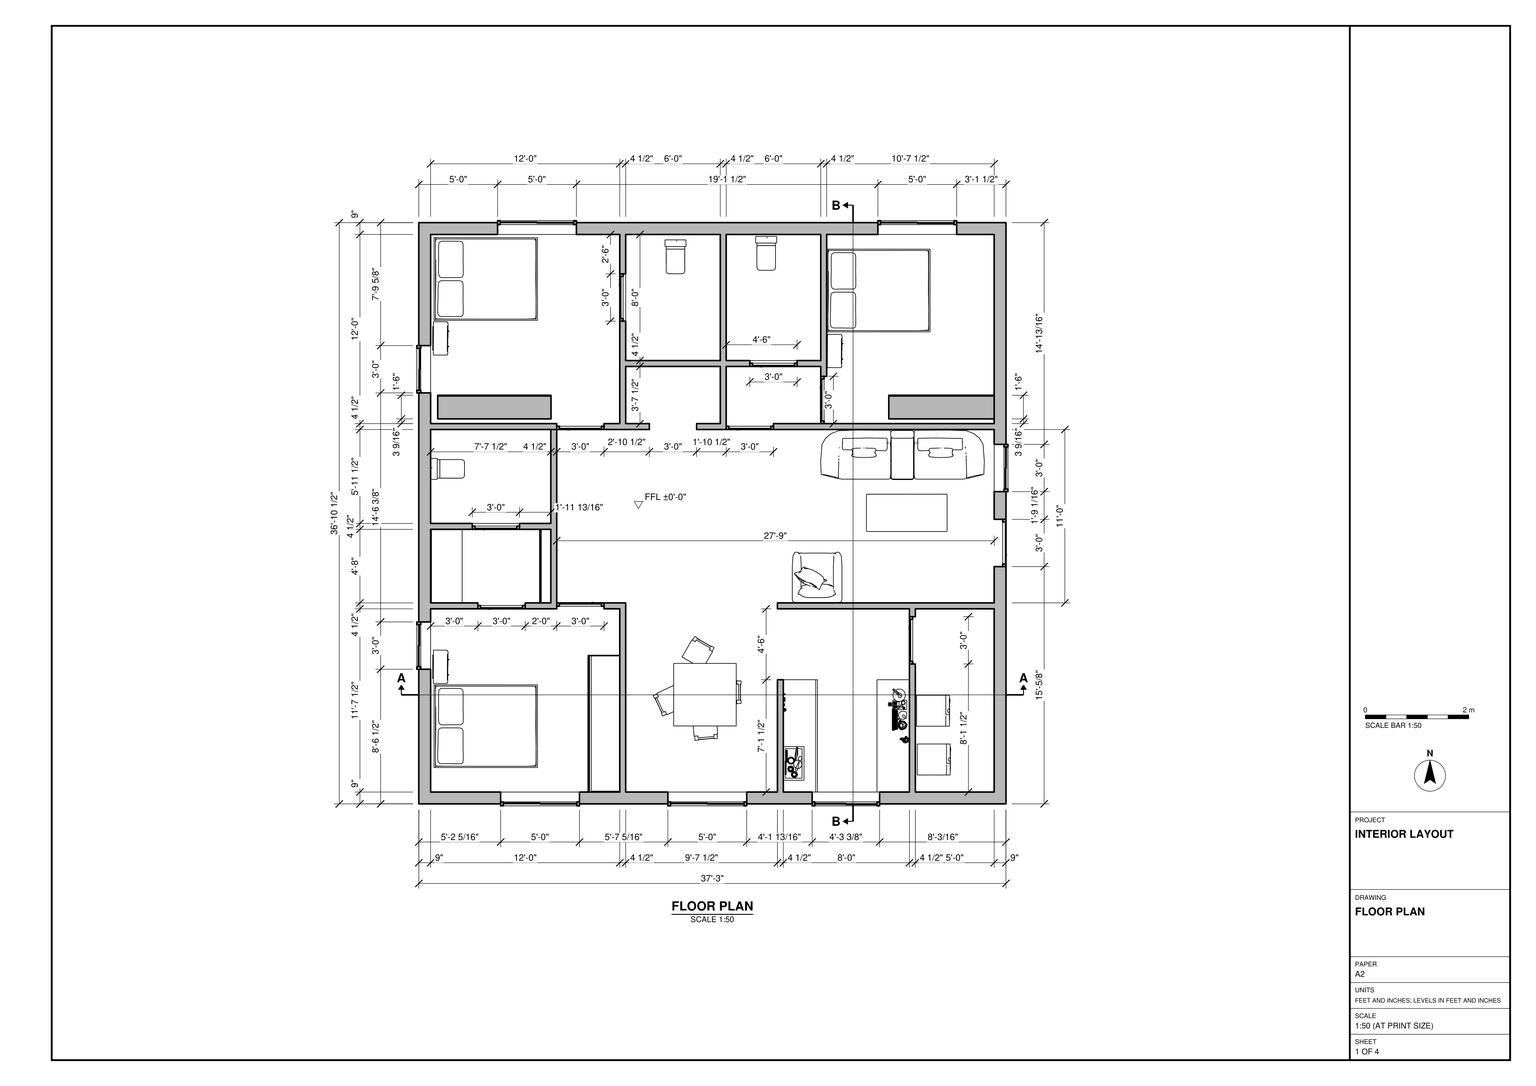
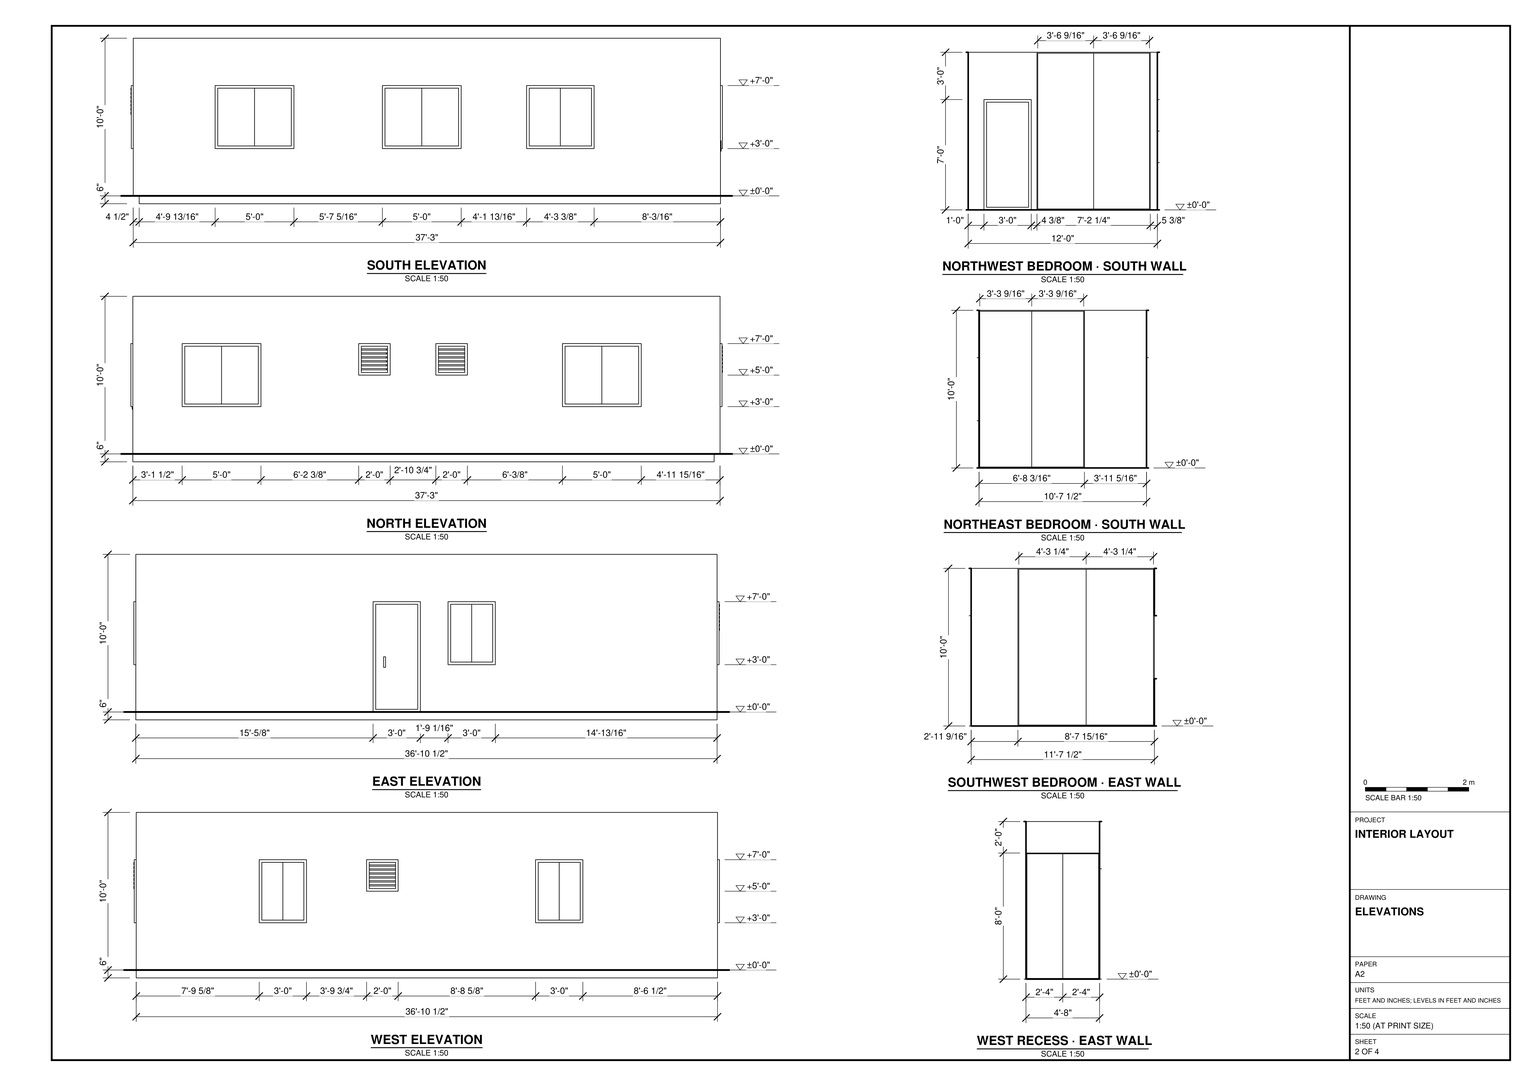
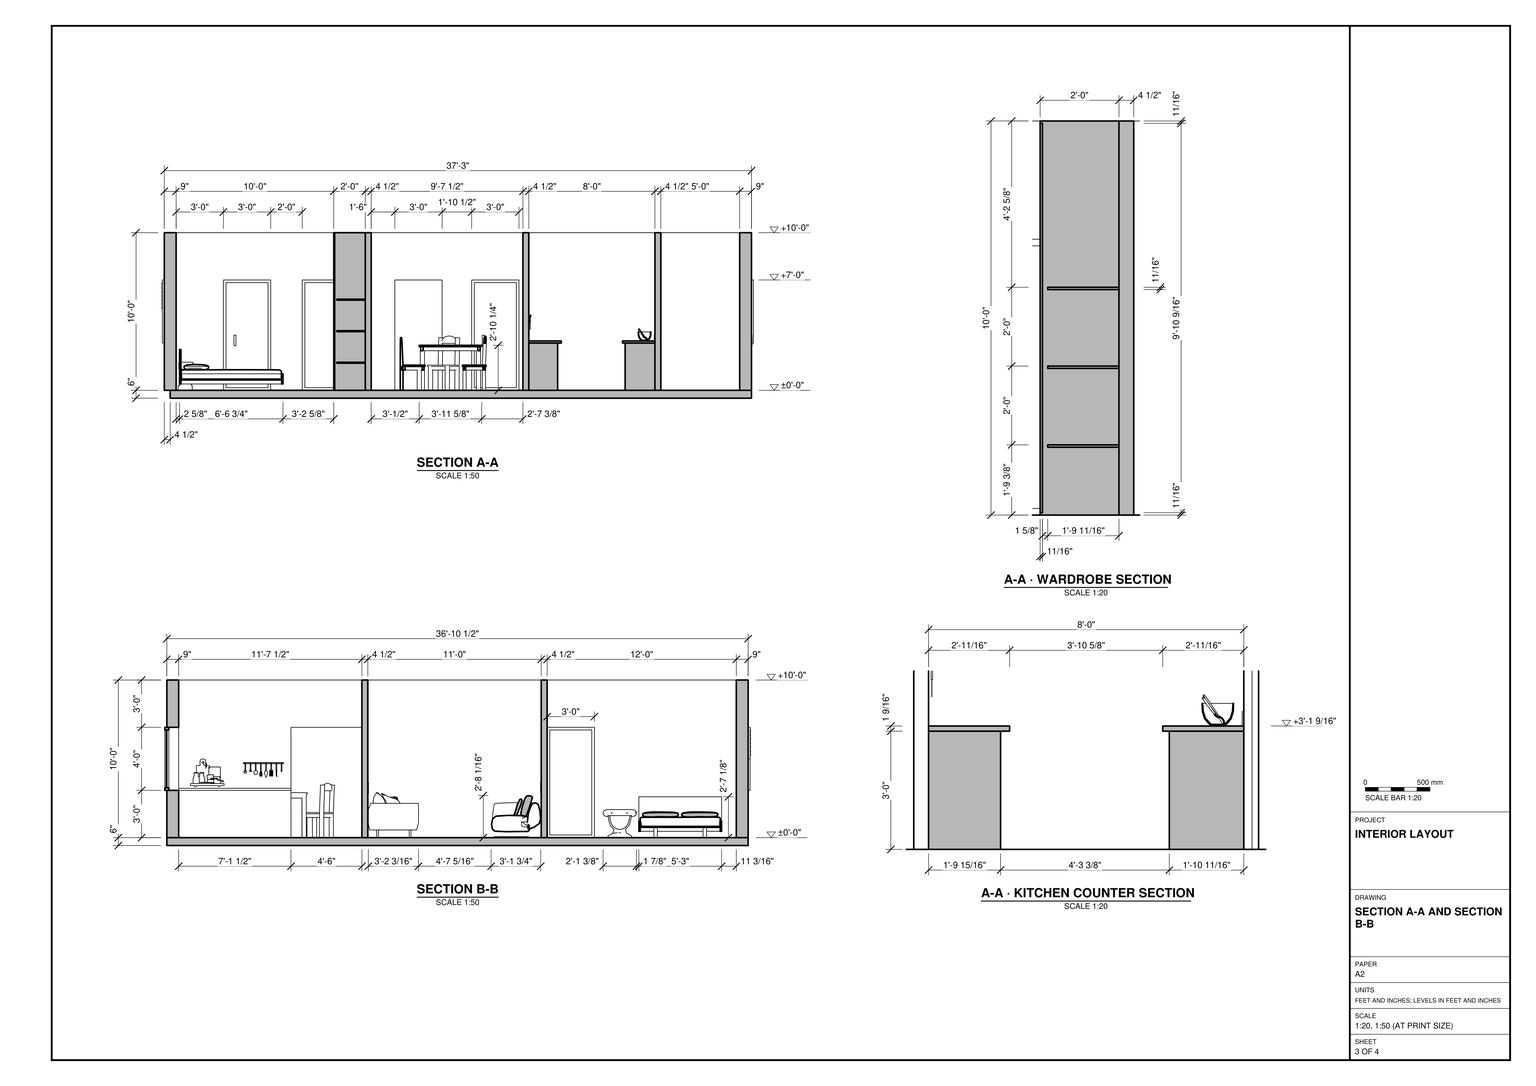
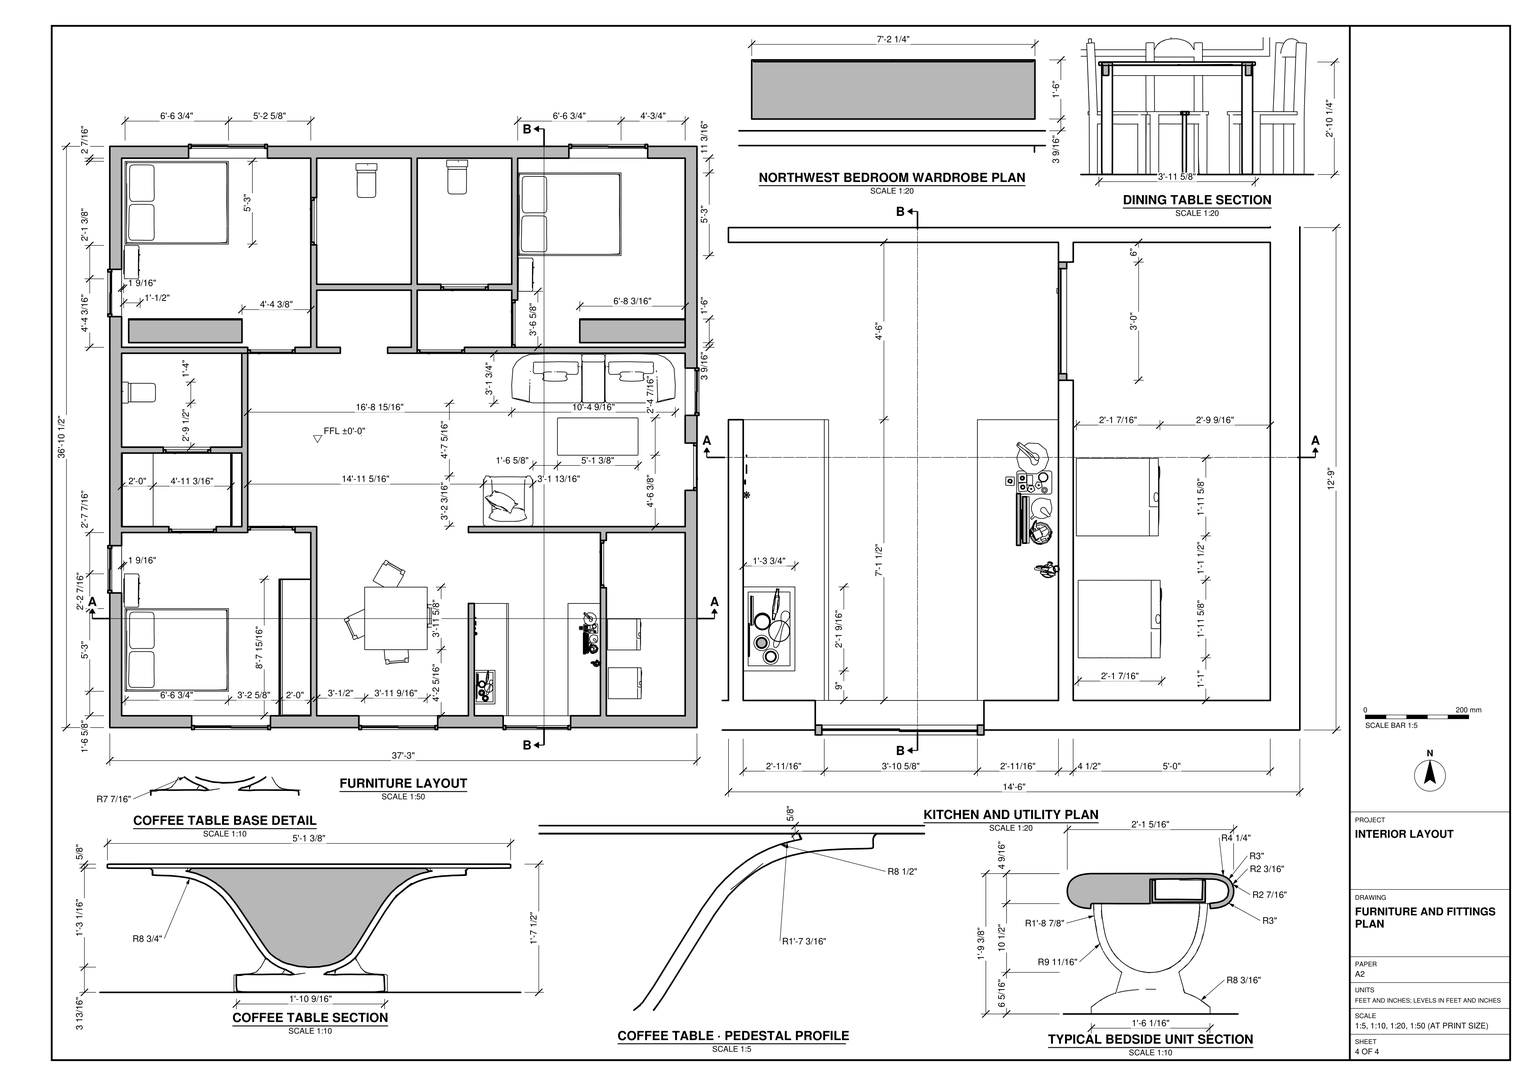
Build the single-storey interior shown in task_files/diagram_01.pdf. Work in feet and inches. Orient the plan with north at the top, east–west along X and north–south along Y. The overall model extents are 37'-6 5/16" along X, 37'-1 13/16" along Y and 10'-6" vertically. Set the finished floor at ±0'-0", with the 6" floor slab below it and the wall tops 10'-0" above it.

Use the plan to lay out the 9" exterior walls and 4 1/2" partitions. Place the bedrooms in the northwest, northeast and southwest corners. Fit the toilet compartments and west recess around the central living space, keeping the passages and doorways as drawn. Use the elevations to position the east entrance, windows and high-level vents.

Furnish the bedrooms with beds, bedside furniture and fitted wardrobes. Follow the interior elevations for the wardrobe widths and the section for the southwest wardrobe shelves. Arrange the sofa, low table and armchair in the eastern living area. Place the dining table and chairs south of the living space, beside the kitchen. Model the two facing kitchen counters with the aisle between them and place the appliances in the adjoining utility space. Decor and loose items, including appliances and kitchen utensils, may be any suitable library components.

Keep the slab, walls, and each furniture or joinery piece in separate groups or components, and use components for repeated parts. Save one SketchUp model as output_files/three_bedroom_interior_with_built_in_wardrobes.skp.

# SketchUp Ruby script. Lengths in inches.
U = 1.inch
M = Sketchup.active_model
def pt(a) = Geom::Point3d.new(a.map { |v| v * U })
def face(e, loops, mat)
  f = e.add_face(loops[0].map { |a| pt(a) })
  loops[1..].each { |l| e.add_face(l.map { |a| pt(a) }).erase! }
  f.material = f.back_material = mat if mat
  f
end
# faces: each face lists its corners as indices into pts; further lists are holes
def faces(e, pts, list, mat = nil) = list.each { |f| face(e, (f[0].is_a?(Array) ? f : [f]).map { |l| l.map { |i| pts[i] } }, mat) }
# xy, xz, yz: faces in a plane at the given z, y or x. An outline is a flat list of corners, or four numbers for a rectangle; further outlines are holes
def ring(l) = l.size == 4 ? [[l[0], l[1]], [l[2], l[1]], [l[2], l[3]], [l[0], l[3]]] : l.each_slice(2).to_a
def flat(e, list, mat, &to3) = list.each { |f| face(e, (f[0].is_a?(Array) ? f : [f]).map { |l| ring(l).map { |u, v| to3.(u, v) } }, mat) }
def xy(e, z, list, mat = nil) = flat(e, list, mat) { |x, y| [x, y, z] }
def xz(e, y, list, mat = nil) = flat(e, list, mat) { |x, z| [x, y, z] }
def yz(e, x, list, mat = nil) = flat(e, list, mat) { |y, z| [x, y, z] }
def lines(e, pts, list) = list.each { |a, b| e.add_line(pt(pts[a]), pt(pts[b])) }
# prism: a flat outline (further loops are holes) pulled along v
def prism(e, loops, v, mat = nil)
  f = face(e, loops, mat); d = Geom::Vector3d.new(v.map { |x| x * U })
  f.pushpull(f.normal.samedirection?(d) ? d.length : -d.length)
end
def box(e, o, s, mat = nil) = prism(e, [[o, [o[0] + s[0], o[1], o[2]], [o[0] + s[0], o[1] + s[1], o[2]], [o[0], o[1] + s[1], o[2]]]], [0, 0, s[2]], mat)
def at(x, y, z, deg = 0) = Geom::Transformation.translation(pt([x, y, z])) * Geom::Transformation.rotation(ORIGIN, Z_AXIS, deg.degrees)
def axes(o, x, y, z) = Geom::Transformation.new([*x, 0, *y, 0, *z, 0, *pt(o).to_a, 1])
def part(name) = M.definitions.add(name)
# library, detail: a bought-in or finely detailed component or shape, given as its bounding box
def library(name, o, s) = part(name).tap { |d| box(d.entities, o, s) }
def detail(e, o, s) = box(e.add_group.entities, o, s)
def put(e, d, t, mat = nil) = e.add_instance(d, t).tap { |i| i.material = mat if mat }
def group(e, t, mat = nil) = e.add_group.tap { |g| g.transformation = t; g.material = mat if mat }.entities
root = M.entities
M.materials.add("Cherry Highgloss 300cm").color = [153, 108, 65]
M.materials.add("Glass Mirror 001").color = [0, 0, 0]
M.materials["Glass Mirror 001"].alpha = 0.1
M.materials.add("Glass Smoked Distorted 001").color = [38, 38, 38]
M.materials["Glass Smoked Distorted 001"].alpha = 0.1
M.materials.add("Marble Black 100cm").color = [32, 32, 32]
M.materials.add("Marble White 100cm").color = [222, 222, 222]
M.materials.add("Metal Sandblasted Black 200cm").color = [86, 90, 95]
M.materials.add("Porcelain SSS 001").color = [245, 243, 236]
M.materials["Porcelain SSS 001"].alpha = 0.6875
M.materials.add("Tiles E 120cm").color = [126, 111, 101]
M.materials.add("Two Color Maple Panels 300cm").color = [56, 46, 41]
M.materials.add("Wall Paint Poised Taupe Satin 300cm").color = [140, 135, 132]
c1 = library("Bed 002",[-31.49,-39.36,0],[62.98,78.72,31.1])
c2 = library("Toy Table Set 40-09",[-39.37,-33.7,0],[66.93,79.21,41.36])
c3 = library("Grad Sofa Set",[-62.1875,-18.88,0],[124.59,37.74,32.07])
c4 = library("Rossi Chair",[-18.9,-19.09,0],[37.8,38.18,34.47])
c5 = library("Table 142 031",[-30.7,-14.21,0],[61.4,28.42,19.53])
c6 = library("Toilet Bowl 127 010",[-8,-12.9,0],[16,25.8,38.91])
c7 = library("Dressing Table 142 024",[-12.69,-6.26,0],[25.38,12.53,21.38])
c8 = library("Kitchen Props 134 014",[-15.6875,-7.04,0],[31.37,14.09,12.97])
c9 = library("Kitchen Utensils 01 92-03",[-3.91,-2.44,0],[7.79,4.85,12.66])
c10 = library("Kitchen Utensils 20-56",[-15.41,-1.59,-10.72],[30.82,2.02,11.3])
c11 = library("Kitchen Utensils Set 92-07",[-12.8,-7.875,0],[25.6,15.75,21.01])
c12 = library("Washer 001",[-11.8125,-12.73,0],[23.63,25.47,33.9])
c13 = part("Group\#32")
box(c13.entities,[0,0,0],[28,0.31,44])
c14 = part("Group\#34")
box(c14.entities,[0,0,0],[28,0.31,44])
c15 = part("Group\#36")
box(c15.entities,[0,0,0],[23.6875,0.31,44])
c16 = part("Group\#38")
box(c16.entities,[-0.31,0,0],[0.31,16,44])
c17 = part("Group\#40")
box(c17.entities,[0,-0.31,0],[28,0.31,44])
c18 = part("Group\#42")
box(c18.entities,[0,0,0],[20,0.31,2])
c19 = part("Group\#44")
box(c19.entities,[0,0,0],[20,0.31,2])
c20 = part("Group\#46")
box(c20.entities,[0,-0.31,0],[28,0.31,44])
c21 = part("Group\#48")
box(c21.entities,[0,0,0],[0.31,16,44])
c22 = part("Group\#50")
box(c22.entities,[-0.31,0,0],[0.31,20,2])
c23 = part("Group\#52")
box(c23.entities,[0,0,0],[0.31,16,44])
c24 = part("Group\#55")
box(c24.entities,[-0.1,0,0],[24.69,85.5,1.57])
p = [[6.31,1.5,0],[1.81,1.5,0]]
lines(root,p,[[0,1]])
put(root,c1,at(52.81,60.64,0,90),"Porcelain SSS 001")
put(root,c1,at(52.81,401.07,0,90),"Porcelain SSS 001")
put(root,c1,at(351.68,392.32,0,90),"Porcelain SSS 001")
put(root,c2,at(219.61,83.46,0),"Porcelain SSS 001")
put(root,c3,at(369.93,267.24,0),"Porcelain SSS 001")
put(root,c4,at(305.05,173.97,0,180),"Porcelain SSS 001")
put(root,c5,at(373.28,223.07,0),"Porcelain SSS 001")
put(root,c6,at(266.27,420.61,0))
put(root,c6,at(197.21,417.96,0))
put(root,c6,at(23.71,256.52,0,90),"Porcelain SSS 001")
put(root,c7,at(18.63,105.86,0,90),"Porcelain SSS 001")
put(root,c7,at(18.63,355.86,0,90),"Porcelain SSS 001")
put(root,c7,at(318.58,346.3,0,90))
put(root,c8,at(366.29,73.43,37.57,90))
put(root,c9,at(371.9,50.28,37.57))
put(root,c10,at(280.91,75.04,56.74,-90))
put(root,c11,at(287.1875,32.29,38.92,90))
put(root,c12,at(394.04,35.29,0,90))
put(root,c12,at(393.48,72.42,0,90))
g1 = group(root,at(6.31,1.5,0))
xy(g1,0,[[[-4.5,0,442.5,0,442.5,180.625,433.5,180.625,433.5,153,268.5,153,268.5,148.5,369,148.5,369,142.5,373.5,142.5,373.5,148.5,433.5,148.5,433.5,9,373.5,9,373.5,106.5,369,106.5,369,9,273,9,273,94.5,299,94.5,299,9,345,9,345,94.5,369,94.5,369,106.5,373.5,106.5,373.5,9,433.5,9,433.5,148.5,373.5,148.5,373.5,142.5,369,142.5,369,148.5,268.5,148.5,268.5,153,433.5,153,433.5,180.625,442.5,180.625,442.5,442.5,-4.5,442.5],[153,337.5,225,433.5],[229.5,337.5,301.5,433.5],[76.5,148.5,76.5,153,96,153,96,209,72.1875,209,72.1875,213.5,96,213.5,96,285,100.5,285,100.5,148.5]]],"Marble White 100cm")
xy(g1,36,[[57.8125,0,117.8125,9],[185.125,0,245.125,9],[294.9375,0,346.3125,9],[-4.5,102.5,4.5,138.5],[433.5,237.6875,442.5,273.6875],
  [-4.5,312.875,4.5,348.875],[55.48,433.5,115.48,442.5],[344.98,433.5,404.98,442.5]],"Wall Paint Poised Taupe Satin 300cm")
xy(g1,60,[[-4.5,243.125,4.5,267.125],[187.85,433.5,211.85,442.5],[246.6,433.5,270.6,442.5]],"Wall Paint Poised Taupe Satin 300cm")
xy(g1,84,[[57.8125,0,117.8125,9],[185.125,0,245.125,9],[294.9375,0,346.3125,9],[268.5,94.5,273,148.5],[-4.5,102.5,4.5,138.5],
  [369,106.5,373.5,142.5],[40.5,148.5,76.5,153],[100.5,148.5,136.5,153],[433.5,180.625,442.5,216.625],[36.1875,209,72.1875,213.5],
  [433.5,237.6875,442.5,273.6875],[-4.5,243.125,4.5,267.125],[100.5,285,136.5,289.5],[171,285,207,289.5],[229.5,285,265.5,289.5],
  [301.5,289.5,306,325.5],[-4.5,312.875,4.5,348.875],[247.5,333,283.5,337.5],[148.5,367.5,153,403.5],[55.48,433.5,115.48,442.5],
  [187.85,433.5,211.85,442.5],[246.6,433.5,270.6,442.5],[344.98,433.5,404.98,442.5]],"Wall Paint Poised Taupe Satin 300cm")
xy(g1,120,[[[-4.5,0,442.5,442.5],[153,9,153,153,100.5,153,100.5,285,96,285,96,213.5,4.5,213.5,4.5,285,433.5,285,433.5,153,268.5,153,268.5,9],[4.5,289.5,148.5,433.5],[4.5,9,148.5,148.5],[306,289.5,433.5,433.5],[273,9,369,148.5],[373.5,9,433.5,148.5],[153,337.5,225,433.5],[229.5,337.5,301.5,433.5],[4.5,153,96,209],[153,289.5,225,333],[229.5,289.5,301.5,333]]],"Wall Paint Poised Taupe Satin 300cm")
xz(g1,0,[[[-4.5,0,442.5,120],[57.8125,36,117.8125,84],[185.125,36,245.125,84],[294.9375,36,346.3125,84]]],"Wall Paint Poised Taupe Satin 300cm")
xz(g1,9,[[[4.5,0,148.5,120],[57.8125,36,117.8125,84]],[[153,0,268.5,120],[185.125,36,245.125,84]],[[273,0,369,120],[294.9375,36,346.3125,84]],[373.5,0,433.5,120]],"Wall Paint Poised Taupe Satin 300cm")
xz(g1,94.5,[[268.5,0,273,84]],"Wall Paint Poised Taupe Satin 300cm")
xz(g1,102.5,[[-4.5,36,4.5,84]],"Wall Paint Poised Taupe Satin 300cm")
xz(g1,106.5,[[369,0,373.5,84]],"Wall Paint Poised Taupe Satin 300cm")
xz(g1,138.5,[[-4.5,36,4.5,84]],"Wall Paint Poised Taupe Satin 300cm")
xz(g1,142.5,[[369,0,373.5,84]],"Wall Paint Poised Taupe Satin 300cm")
xz(g1,148.5,[[4.5,0,40.5,0,40.5,84,76.5,84,76.5,0,100.5,0,100.5,84,136.5,84,136.5,0,148.5,0,148.5,120,4.5,120],[268.5,0,369,0,369,120,273,120,273,84,268.5,84],[373.5,0,433.5,120]],"Wall Paint Poised Taupe Satin 300cm")
xz(g1,153,[[4.5,0,4.5,120,96,120,96,0,76.5,0,76.5,84,40.5,84,40.5,0],[136.5,0,136.5,84,100.5,84,100.5,120,153,120,153,0],[268.5,0,433.5,120]],"Wall Paint Poised Taupe Satin 300cm")
xz(g1,180.625,[[433.5,0,442.5,84]],"Wall Paint Poised Taupe Satin 300cm")
xz(g1,209,[[4.5,0,36.1875,0,36.1875,84,72.1875,84,72.1875,0,96,0,96,120,4.5,120]],"Wall Paint Poised Taupe Satin 300cm")
xz(g1,213.5,[[4.5,0,4.5,120,96,120,96,0,72.1875,0,72.1875,84,36.1875,84,36.1875,0]],"Wall Paint Poised Taupe Satin 300cm")
xz(g1,216.625,[[433.5,0,442.5,84]],"Wall Paint Poised Taupe Satin 300cm")
xz(g1,237.6875,[[433.5,36,442.5,84]],"Wall Paint Poised Taupe Satin 300cm")
xz(g1,243.125,[[-4.5,60,4.5,84]],"Wall Paint Poised Taupe Satin 300cm")
xz(g1,267.125,[[-4.5,60,4.5,84]],"Wall Paint Poised Taupe Satin 300cm")
xz(g1,273.6875,[[433.5,36,442.5,84]],"Wall Paint Poised Taupe Satin 300cm")
xz(g1,285,[[4.5,0,96,120],[96,0,100.5,120],[136.5,0,171,0,171,84,207,84,207,0,229.5,0,229.5,84,265.5,84,265.5,0,433.5,0,433.5,120,100.5,120,100.5,84,136.5,84]],"Wall Paint Poised Taupe Satin 300cm")
xz(g1,289.5,[[4.5,0,4.5,120,148.5,120,148.5,0,136.5,0,136.5,84,100.5,84,100.5,0],[153,0,153,120,225,120,225,0,207,0,207,84,171,84,171,0],[265.5,0,265.5,84,229.5,84,229.5,120,301.5,120,301.5,84,306,84,306,120,433.5,120,433.5,0]],"Wall Paint Poised Taupe Satin 300cm")
xz(g1,312.875,[[-4.5,36,4.5,84]],"Wall Paint Poised Taupe Satin 300cm")
xz(g1,325.5,[[301.5,0,306,84]],"Wall Paint Poised Taupe Satin 300cm")
xz(g1,333,[[153,0,225,120],[229.5,0,247.5,0,247.5,84,283.5,84,283.5,0,301.5,0,301.5,120,229.5,120]],"Wall Paint Poised Taupe Satin 300cm")
xz(g1,337.5,[[153,0,225,120],[229.5,0,229.5,120,301.5,120,301.5,0,283.5,0,283.5,84,247.5,84,247.5,0]],"Wall Paint Poised Taupe Satin 300cm")
xz(g1,348.875,[[-4.5,36,4.5,84]],"Wall Paint Poised Taupe Satin 300cm")
xz(g1,367.5,[[148.5,0,153,84]],"Wall Paint Poised Taupe Satin 300cm")
xz(g1,403.5,[[148.5,0,153,84]],"Wall Paint Poised Taupe Satin 300cm")
xz(g1,433.5,[[[4.5,0,148.5,120],[55.48,36,115.48,84]],[[153,0,225,120],[187.85,60,211.85,84]],[[229.5,0,301.5,120],[246.6,60,270.6,84]],[[306,0,433.5,120],[344.98,36,404.98,84]]],"Wall Paint Poised Taupe Satin 300cm")
xz(g1,442.5,[[[-4.5,0,442.5,120],[344.98,36,404.98,84],[55.48,36,115.48,84],[187.85,60,211.85,84],[246.6,60,270.6,84]]],"Wall Paint Poised Taupe Satin 300cm")
yz(g1,-4.5,[[[0,0,442.5,120],[312.875,36,348.875,84],[102.5,36,138.5,84],[243.125,60,267.125,84]]],"Wall Paint Poised Taupe Satin 300cm")
yz(g1,4.5,[[[9,0,148.5,120],[102.5,36,138.5,84]],[153,0,209,120],[[213.5,0,285,120],[243.125,60,267.125,84]],[[289.5,0,433.5,120],[312.875,36,348.875,84]]],"Wall Paint Poised Taupe Satin 300cm")
yz(g1,36.1875,[[209,0,213.5,84]],"Wall Paint Poised Taupe Satin 300cm")
yz(g1,40.5,[[148.5,0,153,84]],"Wall Paint Poised Taupe Satin 300cm")
yz(g1,55.48,[[433.5,36,442.5,84]],"Wall Paint Poised Taupe Satin 300cm")
yz(g1,57.8125,[[0,36,9,84]],"Wall Paint Poised Taupe Satin 300cm")
yz(g1,72.1875,[[209,0,213.5,84]],"Wall Paint Poised Taupe Satin 300cm")
yz(g1,76.5,[[148.5,0,153,84]],"Wall Paint Poised Taupe Satin 300cm")
yz(g1,96,[[153,0,209,120],[213.5,0,285,120]],"Wall Paint Poised Taupe Satin 300cm")
yz(g1,100.5,[[148.5,0,285,0,285,120,153,120,153,84,148.5,84],[285,0,289.5,84]],"Wall Paint Poised Taupe Satin 300cm")
yz(g1,115.48,[[433.5,36,442.5,84]],"Wall Paint Poised Taupe Satin 300cm")
yz(g1,117.8125,[[0,36,9,84]],"Wall Paint Poised Taupe Satin 300cm")
yz(g1,136.5,[[148.5,0,153,84],[285,0,289.5,84]],"Wall Paint Poised Taupe Satin 300cm")
yz(g1,148.5,[[112.91,0,148.5,120],[289.5,0,289.5,120,433.5,120,433.5,0,403.5,0,403.5,84,367.5,84,367.5,0]],"Wall Paint Poised Taupe Satin 300cm")
yz(g1,153,[[9,0,153,120],[289.5,0,333,120],[337.5,0,367.5,0,367.5,84,403.5,84,403.5,0,433.5,0,433.5,120,337.5,120]],"Wall Paint Poised Taupe Satin 300cm")
yz(g1,171,[[285,0,289.5,84]],"Wall Paint Poised Taupe Satin 300cm")
yz(g1,185.125,[[0,36,9,84]],"Wall Paint Poised Taupe Satin 300cm")
yz(g1,187.85,[[433.5,60,442.5,84]],"Wall Paint Poised Taupe Satin 300cm")
yz(g1,207,[[285,0,289.5,84]],"Wall Paint Poised Taupe Satin 300cm")
yz(g1,211.85,[[433.5,60,442.5,84]],"Wall Paint Poised Taupe Satin 300cm")
yz(g1,225,[[289.5,0,333,120],[337.5,0,433.5,120]],"Wall Paint Poised Taupe Satin 300cm")
yz(g1,229.5,[[285,0,333,0,333,120,289.5,120,289.5,84,285,84],[337.5,0,433.5,120]],"Wall Paint Poised Taupe Satin 300cm")
yz(g1,245.125,[[0,36,9,84]],"Wall Paint Poised Taupe Satin 300cm")
yz(g1,246.6,[[433.5,60,442.5,84]],"Wall Paint Poised Taupe Satin 300cm")
yz(g1,247.5,[[333,0,337.5,84]],"Wall Paint Poised Taupe Satin 300cm")
yz(g1,265.5,[[285,0,289.5,84]],"Wall Paint Poised Taupe Satin 300cm")
yz(g1,268.5,[[9,0,9,120,153,120,153,0,148.5,0,148.5,84,94.5,84,94.5,0]],"Wall Paint Poised Taupe Satin 300cm")
yz(g1,270.6,[[433.5,60,442.5,84]],"Wall Paint Poised Taupe Satin 300cm")
yz(g1,273,[[9,0,94.5,0,94.5,84,148.5,84,148.5,120,9,120]],"Wall Paint Poised Taupe Satin 300cm")
yz(g1,283.5,[[333,0,337.5,84]],"Wall Paint Poised Taupe Satin 300cm")
yz(g1,294.9375,[[0,36,9,84]],"Wall Paint Poised Taupe Satin 300cm")
yz(g1,301.5,[[325.5,0,325.5,84,289.5,84,289.5,120,333,120,333,0],[337.5,0,433.5,120]],"Wall Paint Poised Taupe Satin 300cm")
yz(g1,306,[[325.5,0,433.5,0,433.5,120,289.5,120,289.5,84,325.5,84]],"Wall Paint Poised Taupe Satin 300cm")
yz(g1,344.98,[[433.5,36,442.5,84]],"Wall Paint Poised Taupe Satin 300cm")
yz(g1,346.3125,[[0,36,9,84]],"Wall Paint Poised Taupe Satin 300cm")
yz(g1,369,[[9,0,9,120,148.5,120,148.5,0,142.5,0,142.5,84,106.5,84,106.5,0]],"Wall Paint Poised Taupe Satin 300cm")
yz(g1,373.5,[[9,0,106.5,0,106.5,84,142.5,84,142.5,0,148.5,0,148.5,120,9,120]],"Wall Paint Poised Taupe Satin 300cm")
yz(g1,404.98,[[433.5,36,442.5,84]],"Wall Paint Poised Taupe Satin 300cm")
yz(g1,433.5,[[9,0,148.5,120],[[153,0,153,120,285,120,285,0,216.625,0,216.625,84,180.625,84,180.625,0],[237.6875,36,273.6875,84]],[289.5,0,433.5,120]],"Wall Paint Poised Taupe Satin 300cm")
yz(g1,442.5,[[[0,0,180.625,0,180.625,84,216.625,84,216.625,0,442.5,0,442.5,120,0,120],[237.6875,36,273.6875,84]]],"Wall Paint Poised Taupe Satin 300cm")
g2 = group(g1,at(442.5,180.625,0))
prism(g2,[[[0,0,0],[0,36,0],[0,36,84],[0,0,84]],[[0,34,2],[0,2,2],[0,2,82],[0,34,82]]],[-2.5,0,0],"Metal Sandblasted Black 200cm")
g3 = group(g2,at(0,2,2))
box(g3,[-0.31,0,0],[0.31,32,80],"Two Color Maple Panels 300cm")
g4 = group(g3,at(0,6,32),"Metal Sandblasted Black 200cm")
xy(g4,0,[[0,0,0.5,1.5]])
xy(g4,8,[[0,0,0.5,1.5]])
xz(g4,0,[[0,0,0.5,8]])
xz(g4,1.5,[[0,0,0.5,8]])
yz(g4,0,[[0,0,1.5,8]],"Metal Sandblasted Black 200cm")
yz(g4,0.5,[[0,0,1.5,8]],"Metal Sandblasted Black 200cm")
g5 = group(g1,at(369,106.5,0))
prism(g5,[[[0,0,0],[0,0,84],[0,36,84],[0,36,0]],[[0,2,2],[0,34,2],[0,34,82],[0,2,82]]],[2.5,0,0],"Metal Sandblasted Black 200cm")
g6 = group(g5,at(0,2,2))
xy(g6,0,[[0,0,0.71,32]])
xy(g6,80,[[0,0,0.71,32]])
xz(g6,0,[[0,0,0.71,80]])
xz(g6,32,[[0,0,0.71,80]])
yz(g6,0,[[0,0,32,80]],"Two Color Maple Panels 300cm")
yz(g6,0.71,[[0,0,32,80]])
g7 = group(g6,at(0,26,32),"Metal Sandblasted Black 200cm")
box(g7,[-0.5,-1.5,0],[0.5,1.5,8])
g8 = group(g1,at(100.5,153,0))
prism(g8,[[[0,0,0],[0,0,84],[36,0,84],[36,0,0]],[[34,0,82],[2,0,82],[2,0,2],[34,0,2]]],[0,-2.5,0],"Metal Sandblasted Black 200cm")
g9 = group(g8,at(2,0,2))
box(g9,[0,-0.71,0],[32,0.71,80],"Two Color Maple Panels 300cm")
g10 = group(g9,at(26,0,32),"Metal Sandblasted Black 200cm")
xy(g10,0,[[-1.5,0,0,0.5]])
xy(g10,8,[[-1.5,0,0,0.5]])
xz(g10,0,[[-1.5,0,0,8]],"Metal Sandblasted Black 200cm")
xz(g10,0.5,[[-1.5,0,0,8]],"Metal Sandblasted Black 200cm")
yz(g10,-1.5,[[0,0,0.5,8]])
yz(g10,0,[[0,0,0.5,8]])
g11 = group(g1,at(40.5,148.5,0))
prism(g11,[[[0,0,0],[36,0,0],[36,0,84],[0,0,84]],[[2,0,2],[2,0,82],[34,0,82],[34,0,2]]],[0,2.5,0],"Metal Sandblasted Black 200cm")
g12 = group(g11,at(2,0,2))
box(g12,[0,0,0],[32,0.71,80],"Two Color Maple Panels 300cm")
g13 = group(g12,at(6,0,32),"Metal Sandblasted Black 200cm")
box(g13,[0,-0.5,0],[1.5,0.5,8])
g14 = group(g1,at(36.1875,209,0))
prism(g14,[[[36,0,0],[36,0,84],[0,0,84],[0,0,0]],[[34,0,2],[2,0,2],[2,0,82],[34,0,82]]],[0,2.5,0],"Metal Sandblasted Black 200cm")
g15 = group(g14,at(2,0,2))
box(g15,[0,0,0],[32,0.71,80],"Two Color Maple Panels 300cm")
g16 = group(g15,at(6,0,32),"Metal Sandblasted Black 200cm")
box(g16,[0,-0.5,0],[1.5,0.5,8])
g17 = group(g1,at(100.5,285,0))
prism(g17,[[[36,0,0],[36,0,84],[0,0,84],[0,0,0]],[[34,0,2],[2,0,2],[2,0,82],[34,0,82]]],[0,2.5,0],"Metal Sandblasted Black 200cm")
g18 = group(g17,at(2,0,2),"Two Color Maple Panels 300cm")
xy(g18,0,[[0,0,32,0.71]])
xy(g18,80,[[0,0,32,0.71]])
xz(g18,0,[[0,0,32,80]],"Two Color Maple Panels 300cm")
xz(g18,0.71,[[0,0,32,80]])
yz(g18,0,[[0,0,0.71,80]])
yz(g18,32,[[0,0,0.71,80]])
g19 = group(g18,at(6,0,32),"Metal Sandblasted Black 200cm")
box(g19,[0,-0.5,0],[1.5,0.5,8])
g20 = group(g1,at(229.5,285,0))
prism(g20,[[[36,0,0],[36,0,84],[0,0,84],[0,0,0]],[[2,0,82],[34,0,82],[34,0,2],[2,0,2]]],[0,2.5,0],"Metal Sandblasted Black 200cm")
g21 = group(g20,at(2,0,2))
xy(g21,0,[[0,0,32,0.71]],"Two Color Maple Panels 300cm")
xy(g21,32,[[6,-0.5,7.5,0]],"Two Color Maple Panels 300cm")
xy(g21,40,[[6,-0.5,7.5,0]],"Two Color Maple Panels 300cm")
xy(g21,80,[[0,0,32,0.71]],"Two Color Maple Panels 300cm")
xz(g21,-0.5,[[6,32,7.5,40]],"Two Color Maple Panels 300cm")
xz(g21,0,[[[0,0,32,80],[6,32,7.5,40]]],"Two Color Maple Panels 300cm")
xz(g21,0.71,[[0,0,32,80]],"Two Color Maple Panels 300cm")
yz(g21,0,[[0,0,0.71,80]],"Two Color Maple Panels 300cm")
yz(g21,6,[[-0.5,32,0,40]],"Two Color Maple Panels 300cm")
yz(g21,7.5,[[-0.5,32,0,40]],"Two Color Maple Panels 300cm")
yz(g21,32,[[0,0,0.71,80]],"Two Color Maple Panels 300cm")
g22 = group(g1,at(247.5,333,0))
prism(g22,[[[36,0,0],[36,0,84],[0,0,84],[0,0,0]],[[34,0,82],[34,0,2],[2,0,2],[2,0,82]]],[0,2.5,0],"Metal Sandblasted Black 200cm")
g23 = group(g22,at(2,0,2))
box(g23,[0,0,0],[32,0.71,80],"Two Color Maple Panels 300cm")
g24 = group(g23,at(6,0,32),"Metal Sandblasted Black 200cm")
box(g24,[0,-0.5,0],[1.5,0.5,8])
g25 = group(g1,at(148.5,367.5,0))
prism(g25,[[[0,0,0],[0,0,84],[0,36,84],[0,36,0]],[[0,2,82],[0,2,2],[0,34,2],[0,34,82]]],[2.5,0,0],"Metal Sandblasted Black 200cm")
g26 = group(g25,at(0,2,2))
box(g26,[0,0,0],[0.71,32,80],"Two Color Maple Panels 300cm")
g27 = group(g26,at(0,26,32),"Metal Sandblasted Black 200cm")
box(g27,[-0.5,-1.5,0],[0.5,1.5,8])
g28 = group(g1,at(57.8125,0,36))
prism(g28,[[[0,-1.5,0],[60,-1.5,0],[60,-1.5,48],[0,-1.5,48]],[[58,-1.5,2],[2,-1.5,2],[2,-1.5,46],[58,-1.5,46]]],[0,3,0],"Metal Sandblasted Black 200cm")
put(g28,c13,at(2,0.25,2),"Glass Smoked Distorted 001")
put(g28,c13,at(30,-0.06,2),"Glass Smoked Distorted 001")
g29 = group(g1,at(185.125,0,36))
prism(g29,[[[0,-1.5,0],[60,-1.5,0],[60,-1.5,48],[0,-1.5,48]],[[2,-1.5,2],[2,-1.5,46],[58,-1.5,46],[58,-1.5,2]]],[0,3,0],"Metal Sandblasted Black 200cm")
put(g29,c14,at(2,0.1875,2),"Glass Smoked Distorted 001")
put(g29,c14,at(30,-0.13,2),"Glass Smoked Distorted 001")
g30 = group(g1,at(294.9375,0,36))
prism(g30,[[[0,-1.5,0],[51.375,-1.5,0],[51.375,-1.5,48],[0,-1.5,48]],[[49.375,-1.5,46],[49.375,-1.5,2],[2,-1.5,2],[2,-1.5,46]]],[0,3,0],"Metal Sandblasted Black 200cm")
put(g30,c15,at(2,-0.0625,2),"Glass Smoked Distorted 001")
put(g30,c15,at(25.6875,-0.38,2),"Glass Smoked Distorted 001")
g31 = group(g1,at(442.5,237.6875,36))
prism(g31,[[[1.5,36,0],[1.5,36,48],[1.5,0,48],[1.5,0,0]],[[1.5,34,46],[1.5,34,2],[1.5,2,2],[1.5,2,46]]],[-3,0,0],"Metal Sandblasted Black 200cm")
put(g31,c16,at(-0.1875,2,2),"Glass Smoked Distorted 001")
put(g31,c16,at(0.13,18,2),"Glass Smoked Distorted 001")
g32 = group(g1,at(344.98,442.5,36))
prism(g32,[[[60,1.5,0],[0,1.5,0],[0,1.5,48],[60,1.5,48]],[[2,1.5,2],[58,1.5,2],[58,1.5,46],[2,1.5,46]]],[0,-3,0],"Metal Sandblasted Black 200cm")
put(g32,c17,at(30,-0.125,2),"Glass Smoked Distorted 001")
put(g32,c17,at(2,0.19,2),"Glass Smoked Distorted 001")
g33 = group(g1,at(246.6,442.5,60))
prism(g33,[[[0,1.5,0],[0,1.5,24],[24,1.5,24],[24,1.5,0]],[[2,1.5,22],[2,1.5,2],[22,1.5,2],[22,1.5,22]]],[0,-3,0],"Metal Sandblasted Black 200cm")
put(g33,c18,at(2,1.5,20),"Glass Smoked Distorted 001")
put(g33,c18,at(2,1.5,17),"Glass Smoked Distorted 001")
put(g33,c18,at(2,1.5,14),"Glass Smoked Distorted 001")
put(g33,c18,at(2,1.5,11),"Glass Smoked Distorted 001")
put(g33,c18,at(2,1.5,8),"Glass Smoked Distorted 001")
put(g33,c18,at(2,1.5,5),"Glass Smoked Distorted 001")
put(g33,c18,at(2,1.5,2),"Glass Smoked Distorted 001")
g34 = group(g1,at(187.85,442.5,60))
prism(g34,[[[0,1.5,0],[0,1.5,24],[24,1.5,24],[24,1.5,0]],[[22,1.5,2],[22,1.5,22],[2,1.5,22],[2,1.5,2]]],[0,-3,0],"Metal Sandblasted Black 200cm")
put(g34,c19,at(2,1.5,20),"Glass Smoked Distorted 001")
put(g34,c19,at(2,1.5,17),"Glass Smoked Distorted 001")
put(g34,c19,at(2,1.5,14),"Glass Smoked Distorted 001")
put(g34,c19,at(2,1.5,11),"Glass Smoked Distorted 001")
put(g34,c19,at(2,1.5,8),"Glass Smoked Distorted 001")
put(g34,c19,at(2,1.5,5),"Glass Smoked Distorted 001")
put(g34,c19,at(2,1.5,2),"Glass Smoked Distorted 001")
g35 = group(g1,at(55.48,442.5,36))
prism(g35,[[[60,1.5,0],[0,1.5,0],[0,1.5,48],[60,1.5,48]],[[2,1.5,2],[58,1.5,2],[58,1.5,46],[2,1.5,46]]],[0,-3,0],"Metal Sandblasted Black 200cm")
put(g35,c20,at(30,0.0625,2),"Glass Smoked Distorted 001")
put(g35,c20,at(2,0.38,2),"Glass Smoked Distorted 001")
g36 = group(g1,at(-4.5,312.875,36))
prism(g36,[[[-1.5,36,0],[-1.5,0,0],[-1.5,0,48],[-1.5,36,48]],[[-1.5,2,46],[-1.5,2,2],[-1.5,34,2],[-1.5,34,46]]],[3,0,0],"Metal Sandblasted Black 200cm")
put(g36,c21,at(0.5,18,2),"Glass Smoked Distorted 001")
put(g36,c21,at(0.19,2,2),"Glass Smoked Distorted 001")
g37 = group(g1,at(-4.5,243.125,60))
prism(g37,[[[-1.5,24,0],[-1.5,0,0],[-1.5,0,24],[-1.5,24,24]],[[-1.5,2,2],[-1.5,22,2],[-1.5,22,22],[-1.5,2,22]]],[3,0,0],"Metal Sandblasted Black 200cm")
put(g37,c22,at(-1.5,2,20),"Glass Smoked Distorted 001")
put(g37,c22,at(-1.5,2,17),"Glass Smoked Distorted 001")
put(g37,c22,at(-1.5,2,14),"Glass Smoked Distorted 001")
put(g37,c22,at(-1.5,2,11),"Glass Smoked Distorted 001")
put(g37,c22,at(-1.5,2,8),"Glass Smoked Distorted 001")
put(g37,c22,at(-1.5,2,5),"Glass Smoked Distorted 001")
put(g37,c22,at(-1.5,2,2),"Glass Smoked Distorted 001")
g38 = group(g1,at(-4.5,102.5,36))
prism(g38,[[[-1.5,36,0],[-1.5,0,0],[-1.5,0,48],[-1.5,36,48]],[[-1.5,34,2],[-1.5,34,46],[-1.5,2,46],[-1.5,2,2]]],[3,0,0],"Metal Sandblasted Black 200cm")
put(g38,c23,at(0.0625,18,2),"Glass Smoked Distorted 001")
put(g38,c23,at(-0.25,2,2),"Glass Smoked Distorted 001")
g39 = group(g1,at(345,9,0),"Cherry Highgloss 300cm")
box(g39,[1.3125,0,0],[22.6875,85.5,36],"Cherry Highgloss 300cm")
g40 = group(g1,at(273,9,0),"Cherry Highgloss 300cm")
box(g40,[0,0,0],[21.9375,85.5,36],"Cherry Highgloss 300cm")
g41 = group(g1,at(346.3125,9,36))
xy(g41,0,[[0,0,22.6875,85.5]])
put(g1,c24,at(344.41,9,36),"Marble Black 100cm")
put(g1,c24,at(273.1,9,36),"Marble Black 100cm")
g42 = group(g1,at(301.5,289.5,0))
prism(g42,[[[0,36,84],[0,36,0],[0,0,0],[0,0,84]],[[0,2,2],[0,34,2],[0,34,82],[0,2,82]]],[2.5,0,0],"Metal Sandblasted Black 200cm")
g43 = group(g42,at(0,2,2),"Two Color Maple Panels 300cm")
xy(g43,0,[[0,0,0.71,32]])
xy(g43,80,[[0,0,0.71,32]])
xz(g43,0,[[0,0,0.71,80]])
xz(g43,32,[[0,0,0.71,80]])
yz(g43,0,[[0,0,32,80]],"Two Color Maple Panels 300cm")
yz(g43,0.71,[[0,0,32,80]])
g44 = group(g43,at(0,26,32),"Metal Sandblasted Black 200cm")
box(g44,[-0.5,-1.5,0],[0.5,1.5,8])
g45 = group(g1,at(148.5,9,0),"Cherry Highgloss 300cm")
box(g45,[-24,0,0],[24,103.91,120],"Cherry Highgloss 300cm")
g46 = group(g45,at(-24,0.71,-2.98))
box(g46,[2.3125,0,23.65],[21.6875,103.2,0.7],"Cherry Highgloss 300cm")
g47 = group(g45,at(-24,0.71,21.02))
box(g47,[2.3125,0,23.65],[21.6875,103.2,0.7],"Cherry Highgloss 300cm")
g48 = group(g45,at(-24,0.71,45.02))
box(g48,[2.3125,0,23.65],[21.6875,103.2,0.7],"Cherry Highgloss 300cm")
g49 = group(g45,at(-24,51.96,0.71))
box(g49,[0,0,0],[0.71,51.25,118.58],"Cherry Highgloss 300cm")
g50 = group(g45,at(-24,0.71,0.71))
box(g50,[0,0,0],[0.71,51.25,118.58],"Cherry Highgloss 300cm")
g51 = group(g1,at(9.9,293.08,0),"Cherry Highgloss 300cm")
box(g51,[0,0,0],[86.25,18,120],"Cherry Highgloss 300cm")
g52 = group(g51,at(0.59,18,-2.98))
box(g52,[0,-18,23.65],[85.66,16.27,0.7],"Cherry Highgloss 300cm")
g53 = group(g51,at(0.59,18,21.02))
box(g53,[0,-18,23.65],[85.66,16.27,0.7],"Cherry Highgloss 300cm")
g54 = group(g51,at(0.59,18,45.02))
box(g54,[0,-18,23.65],[85.66,16.27,0.7],"Cherry Highgloss 300cm")
g55 = group(g51,at(43.125,18,0.71))
box(g55,[0,-0.53,0],[42.53,0.53,118.58],"Cherry Highgloss 300cm")
g56 = group(g51,at(0.59,18,0.71))
box(g56,[0,-0.53,0],[42.53,0.53,118.58],"Cherry Highgloss 300cm")
g57 = group(g1,at(353.29,293.08,0),"Cherry Highgloss 300cm")
box(g57,[0,0,0],[80.21,18,120],"Cherry Highgloss 300cm")
g58 = group(g57,at(0.55,18,-2.98))
box(g58,[0,-18,23.65],[79.66,16.27,0.7],"Cherry Highgloss 300cm")
g59 = group(g57,at(0.55,18,21.02))
box(g59,[0,-18,23.65],[79.66,16.27,0.7],"Cherry Highgloss 300cm")
g60 = group(g57,at(0.55,18,45.02))
box(g60,[0,-18,23.65],[79.66,16.27,0.7],"Cherry Highgloss 300cm")
g61 = group(g57,at(40.1,18,0.71))
box(g61,[0,-0.53,0],[39.56,0.53,118.58],"Cherry Highgloss 300cm")
g62 = group(g57,at(0.55,18,0.71))
box(g62,[0,-0.53,0],[39.56,0.53,118.58],"Cherry Highgloss 300cm")
g63 = group(g1,at(153,337.5,0))
xy(g63,0,[[0,0,72,96]],"Tiles E 120cm")
g64 = group(g1,at(229.5,337.5,0))
xy(g64,0,[[0,0,72,96]],"Tiles E 120cm")
g65 = group(root,at(6.31,1.5,0))
xy(g65,-6,[[0,0,442.5,442.5]])
xy(g65,0,[[273,9,299,94.5],[345,9,369,94.5]])
xz(g65,0,[[0,-6,442.5,0]])
xz(g65,442.5,[[0,-6,442.5,0]])
yz(g65,0,[[0,-6,442.5,0]])
yz(g65,442.5,[[0,-6,442.5,0]])
g66 = group(root,at(10.81,154.5,0))
box(g66,[0,0,0],[24,56,36],"Cherry Highgloss 300cm")
g67 = group(root,at(10.81,154.5,36),"Glass Mirror 001")
box(g67,[0,0,0],[0.31,56,84],"Glass Mirror 001")
g68 = group(root,at(82.81,154.5,0),"Cherry Highgloss 300cm")
xy(g68,0,[[11.1875,0,19.5,56]],"Cherry Highgloss 300cm")
xy(g68,96,[[11.1875,0,19.5,56]],"Cherry Highgloss 300cm")
xz(g68,0,[[11.1875,0,19.5,96]],"Cherry Highgloss 300cm")
xz(g68,56,[[11.1875,0,19.5,96]],"Cherry Highgloss 300cm")
yz(g68,11.1875,[[[0.1,0.08,55.9,95.92],[0.71,0.57,55.29,95.43]]],"Cherry Highgloss 300cm")
yz(g68,19.5,[[0,0,56,96]],"Cherry Highgloss 300cm")
g69 = group(g68,at(11.1875,28,0.57))
box(g69,[0,0,0],[0.71,27.29,94.87],"Cherry Highgloss 300cm")
g70 = group(g68,at(11.1875,0.71,0.57))
box(g70,[0,0,0],[0.71,27.29,94.87],"Cherry Highgloss 300cm")
g71 = group(root,at(10.81,215,0))
box(g71,[0,0,0],[91.5,71.5,0.2],"Tiles E 120cm")
